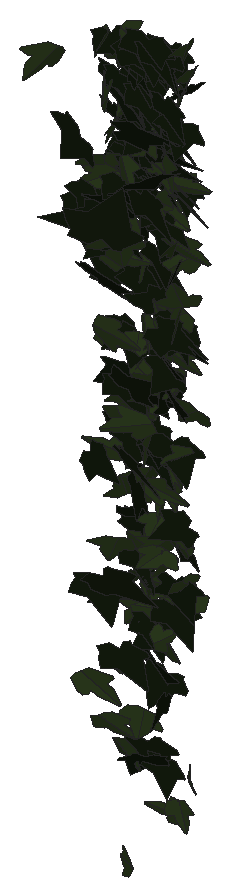
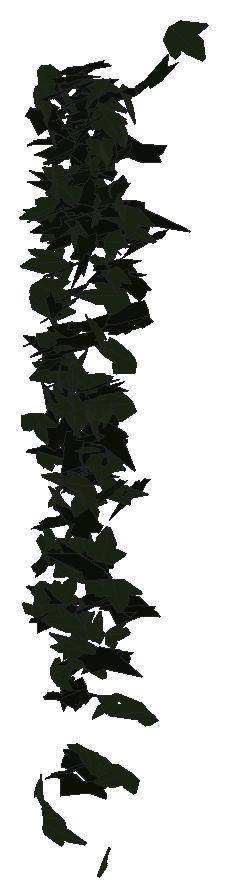
# SketchUp Ruby script. Lengths in millimetres.
U = 1.mm
M = Sketchup.active_model
def pt(a) = Geom::Point3d.new(a.map { |v| v * U })
def face(e, loops, mat)
  f = e.add_face(loops[0].map { |a| pt(a) })
  loops[1..].each { |l| e.add_face(l.map { |a| pt(a) }).erase! }
  f.material = f.back_material = mat if mat
  f
end
# faces: each face lists its corners as indices into pts; further lists are holes
def faces(e, pts, list, mat = nil) = list.each { |f| face(e, (f[0].is_a?(Array) ? f : [f]).map { |l| l.map { |i| pts[i] } }, mat) }
# xy, xz, yz: faces in a plane at the given z, y or x. An outline is a flat list of corners, or four numbers for a rectangle; further outlines are holes
def ring(l) = l.size == 4 ? [[l[0], l[1]], [l[2], l[1]], [l[2], l[3]], [l[0], l[3]]] : l.each_slice(2).to_a
def flat(e, list, mat, &to3) = list.each { |f| face(e, (f[0].is_a?(Array) ? f : [f]).map { |l| ring(l).map { |u, v| to3.(u, v) } }, mat) }
def xy(e, z, list, mat = nil) = flat(e, list, mat) { |x, y| [x, y, z] }
def xz(e, y, list, mat = nil) = flat(e, list, mat) { |x, z| [x, y, z] }
def yz(e, x, list, mat = nil) = flat(e, list, mat) { |y, z| [x, y, z] }
def lines(e, pts, list) = list.each { |a, b| e.add_line(pt(pts[a]), pt(pts[b])) }
# prism: a flat outline (further loops are holes) pulled along v
def prism(e, loops, v, mat = nil)
  f = face(e, loops, mat); d = Geom::Vector3d.new(v.map { |x| x * U })
  f.pushpull(f.normal.samedirection?(d) ? d.length : -d.length)
end
def box(e, o, s, mat = nil) = prism(e, [[o, [o[0] + s[0], o[1], o[2]], [o[0] + s[0], o[1] + s[1], o[2]], [o[0], o[1] + s[1], o[2]]]], [0, 0, s[2]], mat)
def at(x, y, z, deg = 0) = Geom::Transformation.translation(pt([x, y, z])) * Geom::Transformation.rotation(ORIGIN, Z_AXIS, deg.degrees)
def axes(o, x, y, z) = Geom::Transformation.new([*x, 0, *y, 0, *z, 0, *pt(o).to_a, 1])
def part(name) = M.definitions.add(name)
# library, detail: a bought-in or finely detailed component or shape, given as its bounding box
def library(name, o, s) = part(name).tap { |d| box(d.entities, o, s) }
def detail(e, o, s) = box(e.add_group.entities, o, s)
def put(e, d, t, mat = nil) = e.add_instance(d, t).tap { |i| i.material = mat if mat }
def group(e, t, mat = nil) = e.add_group.tap { |g| g.transformation = t; g.material = mat if mat }.entities
root = M.entities
M.materials.add("efeu1").color = [18, 25, 13]
M.materials.add("efeu2").color = [43, 57, 29]
c1 = part("ivyleaf_9")
p = [[39.1,54.8,31.7],[34.5,51.8,30.2],[-5.3,25.2,17.3],[-17.9,28.3,20.9],[-21.6,21.7,17],[-20.2,4.3,5.3],
  [-22.9,-0.3,2.5],[-17.1,-4,-0.6],[-2,-2.1,-1.2],[-0.7,-15.4,-10.1],[16.6,-22.3,-16.7],[21.1,-15.1,-12.5],
  [32.7,-10.7,-11],[46.1,-1.8,-6.6],[30.8,11.2,3.8]]
faces(c1.entities,p,[[0,1,2,3,4,5,6,7,8,9,10,11,12,13,14]],"efeu1")
c2 = part("ivyleaf_10")
p = [[0,12.8,-0.8],[-1.5,51.3,-10.9],[-4.9,51,-11.6],[-13.6,26.5,-7.3],[-13.2,15.9,-4.6],[-21.1,19.3,-7.2],
  [-29.5,16.3,-8.3],[-29.2,8.3,-6.2],[-19.7,-9.8,0.5],[-7.6,-13,4],[1,-12.2,5.8],[-0.4,51.1,-11.1],
  [-1.5,51.1,-10.9],[1,-12.4,5.9],[16.9,-12.4,3.5],[35.1,9.1,-5.1],[35,12.9,-6.1],[20.5,16.4,-4.9],
  [15.8,15,-3.8],[15.3,27.6,-7.1],[12.8,31.3,-7.8]]
faces(c2.entities,p,[[0,1,2,3,4,5,6,7,8,9,10],[11,12,0,13,14,15,16,17,18,19,20]],"efeu2")
put(root,c1,axes([2025,744.4,1522.4],[-0.59045,-0.57511,0.96356],[-0.27948,-0.9703,-0.62642],[2.11729,-0.28846,0.18602]))
put(root,c1,axes([2083.3,733,1360.2],[-1.5486,-0.12856,0.81863],[1.53227,0.14899,0.82363],[-0.3734,1.14456,-0.01526]))
put(root,c2,axes([1950.2,760.7,1650.6],[-0.45254,-0.90858,0.68289],[-0.14048,-0.68385,-0.93556],[2.1586,-0.23498,0.08228]))
put(root,c1,axes([2027.4,832.8,1321.6],[-0.43087,-0.35158,-0.98103],[-1.10797,-0.79,0.41746],[-1.64506,0.62416,-0.02422]))
put(root,c2,axes([2084.4,834.2,963],[-0.61889,-0.15247,0.84845],[-1.00894,-0.67969,-0.32533],[1.29371,-0.60302,0.15216]))
put(root,c2,axes([2044.6,827.3,1294.8],[-1.29698,-0.81371,-0.15005],[0.18292,0.11523,-1.06138],[1.56411,-0.68822,-0.0003]))
put(root,c1,axes([2039.7,842.7,887.6],[1.06306,-0.71655,0.03403],[0.04076,-0.02645,-0.90854],[1.36467,0.55898,0.00063]))
put(root,c1,axes([2094.1,823.6,1427.4],[0.72709,0.98395,0.23303],[0.16081,0.21717,-1.05551],[-1.91772,0.39127,-0.00016]))
put(root,c1,axes([2050.2,864.7,822.7],[0.41731,-0.17934,-0.93924],[1.34399,-0.61934,0.28311],[-1.22702,-0.73937,-0.00933]))
put(root,c1,axes([1950.7,881.2,1323.8],[-0.66445,-0.72966,0.43215],[-0.13711,-0.44014,-0.80134],[1.60814,-0.339,0.11024]))
put(root,c1,axes([2058.5,871,1365.5],[0.5974,-0.8535,-0.21236],[-0.09904,0.20706,-0.90912],[1.67097,0.31741,0.02204]))
put(root,c1,axes([1927.1,869.4,1315.7],[0.29792,-0.80255,-0.41602],[-0.13796,0.40971,-0.81765],[1.71489,0.17239,0.0065]))
put(root,c2,axes([2021.4,870.1,1414.8],[-0.08495,0.88501,-0.17145],[0.01922,-0.17115,-0.88614],[-1.71556,-0.04574,-0.00144]))
put(root,c1,axes([1959.6,881.1,598.4],[-0.64268,-0.70628,-0.39631],[0.3504,0.35119,-0.78275],[1.50099,-0.38439,0.01304]))
put(root,c1,axes([2006.1,877.2,490],[-0.10418,-0.68227,-0.5508],[0.1789,0.54413,-0.68334],[1.65921,-0.10151,0.0391]))
put(root,c2,axes([1964.7,886.5,1077],[-0.06447,0.03819,-0.96645],[1.52583,-0.53985,-0.04943],[-1.02973,-0.80233,-0.01274]))
put(root,c1,axes([1972.1,888.6,1309.1],[1.88697,0.26607,0.22449],[-0.42479,-0.03415,1.02627],[0.50845,-1.016,0.02429]))
put(root,c2,axes([2011,891.6,79.2],[-0.5212,0.5755,0.41446],[0.32636,-0.37737,0.6373],[1.30971,0.32305,0.00613]))
put(root,c2,axes([1932.9,882.9,408.6],[0.95655,0.17501,0.67755],[1.22317,0.21461,-0.53218],[-0.52695,0.81586,-0.00536]))
put(root,c1,axes([1974.9,877.5,616.7],[-0.00616,-0.09918,-0.87578],[0.74471,0.78459,-0.0903],[1.50308,-0.38914,0.04115]))
put(root,c1,axes([1942.5,898,1160.1],[0.00503,-0.4091,0.7989],[1.07046,-0.62183,-0.32029],[1.33122,0.50157,0.25453]))
put(root,c1,axes([1943.4,881,837],[0.55134,-0.5067,-0.76251],[-0.70629,0.66613,-0.58364],[1.59285,0.47076,0.00513]))
put(root,c1,axes([2078.3,903.6,410.2],[-0.26455,0.19758,-0.73243],[0.88609,-0.56567,-0.24095],[-1.13989,-0.48558,-0.01732]))
put(root,c1,axes([1988.6,912.6,1497.6],[-0.39767,-0.43201,0.83597],[0.22129,-0.86162,-0.4162],[1.77719,0.01062,0.23888]))
put(root,c1,axes([1998,896.9,1363.8],[-0.07585,-0.80628,-0.50177],[0.04979,0.50109,-0.80726],[1.8067,-0.04766,0.00118]))
put(root,c1,axes([1971.6,908.8,1244.4],[-1.05319,-0.49747,0.25851],[-0.3625,-0.17479,-0.74411],[1.00351,-0.58524,0.00251]))
put(root,c2,axes([2060.2,897.9,805.6],[0.19964,0.03854,0.74126],[1.38352,0.14594,-0.11046],[-0.28545,0.73428,-0.01695]))
put(root,c1,axes([2039.6,898.7,289.4],[0.44416,0.62056,-0.38436],[-0.26488,-0.3583,-0.66299],[-1.36377,0.2717,0.00359]))
put(root,c2,axes([1984.8,907.6,291.2],[-0.83427,0.37906,-0.48542],[0.68928,-0.32326,-0.57949],[-0.94808,-0.56858,0.00585]))
put(root,c2,axes([2034.4,918,879.4],[0.38125,-0.68078,0.51492],[0.50201,-0.45365,-0.70239],[1.54503,0.31539,0.10116]))
put(root,c1,axes([1991.4,904.1,1452.1],[1.02445,0.21175,-0.63507],[0.98202,0.38797,0.56669],[0.81175,-0.73657,0.11592]))
put(root,c2,axes([1952.6,915.1,1352.3],[0.8859,0.32847,-0.70126],[-1.17258,-0.33857,-0.56755],[-0.89281,0.77059,0.04956]))
put(root,c2,axes([1962.1,891.5,1508.9],[0.44742,-0.28858,0.96722],[-1.10044,0.77551,0.37192],[-1.57456,-0.62399,0.01491]))
put(root,c1,axes([2068.1,918.1,1527.4],[0.35814,-0.82673,0.10934],[0.03484,-0.10797,-0.84786],[1.58676,0.18897,-0.00606]))
put(root,c1,axes([2031.3,919.3,1628.5],[-0.40377,-0.90102,-0.1024],[0.04736,0.09934,-0.92566],[1.7252,-0.2136,0.00145]))
put(root,c2,axes([2094.1,907.8,1272.6],[0.01395,-0.75862,-0.2512],[-0.01958,0.2511,-0.75862],[1.52078,0.01019,-0.00746]))
put(root,c1,axes([2071.2,900.5,1106.8],[0.61999,-0.40309,-0.77176],[-0.09407,0.81412,-0.44608],[1.65442,0.19735,0.26385]))
put(root,c2,axes([1970.1,916.2,835.1],[0.37409,0.13798,0.69312],[-1.09664,-0.38526,0.2401],[0.77877,-0.60879,0.00515]))
put(root,c2,axes([1958.6,928.4,566.7],[-0.29916,-0.20614,0.77495],[0.24086,-0.78618,-0.18346],[1.50705,0.08473,0.18315]))
put(root,c1,axes([2028.9,930.1,857],[-0.15017,-0.48877,0.70375],[0.26647,-0.70458,-0.47365],[1.60879,0.07108,0.14414]))
put(root,c1,axes([2036.5,919.8,1616],[0.44568,-0.82718,-0.10521],[-0.00875,0.10799,-0.85933],[1.58695,0.2329,0.02481]))
put(root,c1,axes([2068.4,931.5,1015.1],[-0.65818,-0.60775,0.4634],[-0.24148,-0.45592,-0.69263],[1.43436,-0.35563,0.09603]))
put(root,c1,axes([2101.4,930.2,731.4],[-0.80179,-0.39468,0.56978],[-0.71924,-0.42814,-0.57599],[1.10581,-0.56464,0.03849]))
put(root,c1,axes([2039.2,932.5,1321.7],[-0.69848,-0.62396,0.42429],[-0.08492,-0.45304,-0.70484],[1.43355,-0.33085,0.16498]))
put(root,c2,axes([2069.8,901.9,1347.5],[-0.08237,0.48159,0.64392],[-0.31237,0.62599,-0.47921],[-1.49813,-0.157,0.06451]))
put(root,c1,axes([1987.6,923.2,954.9],[-0.47855,0.02371,0.8195],[0.88765,-0.70082,0.16338],[1.28324,0.49362,0.1926]))
put(root,c2,axes([1936.8,921,1606.5],[0.53239,-0.8435,0.02444],[0.015,-0.02313,-0.88868],[1.60596,0.27984,0.0002]))
put(root,c2,axes([1941.1,915.8,1377],[-1.12336,-0.66652,-0.1353],[0.18086,0.09656,-0.89027],[1.28169,-0.59781,0.00704]))
put(root,c2,axes([1987.3,920.5,1601.8],[-0.07017,-0.89126,0.02368],[-0.00471,-0.0236,-0.89203],[1.69685,-0.03692,-0.0015]))
put(root,c1,axes([2058,929.1,271.6],[-0.28259,-0.76576,0.05285],[-0.03019,-0.05076,-0.78],[1.46055,-0.14921,-0.0059]))
put(root,c1,axes([1933.8,919,1263.4],[-0.40067,-0.10092,-0.86869],[1.44649,0.42089,-0.23309],[0.82336,-0.78854,-0.01324]))
put(root,c1,axes([2012.5,927.5,1521.6],[0.11998,-0.8391,-0.12858],[-0.00001,0.12893,-0.84142],[1.61562,0.06231,0.00955]))
put(root,c2,axes([2097.8,933.2,866.1],[-0.09863,-0.31934,0.67271],[-0.32182,-0.65167,-0.32238],[1.38021,-0.17477,-0.02709]))
put(root,c2,axes([2083.5,930.4,1127.9],[0.72712,-0.74233,0.4175],[0.46151,-0.34383,-0.83325],[1.55384,0.4495,0.05212]))
put(root,c2,axes([1965,910.8,1209.7],[-0.29853,-0.14478,-0.90391],[1.53988,0.40706,-0.20561],[0.81498,-0.82216,0.05738]))
put(root,c1,axes([1996,917.5,1610.3],[0.30379,-0.61305,-0.58444],[-0.03631,0.59197,-0.62616],[1.61158,0.1289,0.09606]))
put(root,c2,axes([2047.1,929,1403.9],[1.19859,-0.31022,0.57392],[1.01111,-0.21911,-0.70141],[0.72063,0.8234,0.02958]))
put(root,c2,axes([1959.8,923.8,658.2],[-1.07767,-0.593,0.10866],[-0.12819,-0.08591,-0.81986],[1.1402,-0.57014,0.01053]))
put(root,c1,axes([2068.5,936.2,955.5],[0.11624,-0.26606,0.77227],[0.34211,-0.75106,-0.27297],[1.51646,0.18983,0.00239]))
put(root,c1,axes([1965.5,930.4,1539.1],[0.20927,-0.84086,-0.06432],[-0.02125,0.06341,-0.84802],[1.60486,0.11048,-0.00284]))
put(root,c1,axes([2076.4,928.8,881.7],[-0.58486,-0.7536,-0.39936],[0.30652,0.36559,-0.81379],[1.594,-0.34681,0.00995]))
put(root,c2,axes([2048.1,929.5,663.4],[0.98136,0.31871,-0.46657],[-0.75333,-0.24702,-0.60618],[-0.76742,0.65004,-0.0016]))
put(root,c1,axes([2048.7,938.5,1609.9],[-0.87267,-0.67369,0.15156],[-0.07103,-0.15748,-0.81295],[1.31229,-0.45653,0.05678]))
put(root,c1,axes([1950.5,927.1,1609.6],[0.07191,-0.81992,-0.44115],[-0.05258,0.44033,-0.82077],[1.77122,0.04636,-0.00645]))
put(root,c2,axes([2017.6,930.7,1090.2],[-0.10176,0.80361,-0.41174],[0.0647,-0.41038,-0.80536],[-1.71727,-0.06308,-0.00594]))
put(root,c1,axes([2039.6,936.2,1597.6],[0.43029,-0.81824,0.17506],[0.06703,-0.17187,-0.84882],[1.5911,0.22852,-0.01158]))
put(root,c2,axes([2047.1,933.9,682.9],[-0.67321,-0.58412,0.4179],[-0.41833,-0.35544,-0.68287],[1.30132,-0.41644,-0.00333]))
put(root,c2,axes([1956.3,942.6,1283.9],[0.03091,-0.00866,-0.82731],[0.00883,-0.82745,0.00875],[-1.57459,-0.00481,-0.01619]))
put(root,c1,axes([2003,938.7,860.7],[-0.86184,-0.61602,0.09287],[-0.07741,-0.08533,-0.76435],[1.18313,-0.45432,0.01764]))
put(root,c1,axes([2087.2,940.3,1480.8],[-0.58709,-0.78065,0.13568],[-0.06691,-0.13197,-0.83924],[1.50652,-0.31008,0.0156]))
put(root,c2,axes([2015.1,926.3,1590.9],[-0.12042,0.00925,0.89983],[-1.70221,-0.10006,-0.06186],[0.18876,-0.89648,0.01619]))
put(root,c2,axes([2013.4,927.9,1433.5],[1.32658,-0.3506,-0.20457],[-0.32602,0.11448,-0.77985],[0.70039,0.71735,0.02447]))
put(root,c2,axes([1966.3,931.1,1273.6],[1.58491,-0.33134,-0.01417],[-0.02655,0.00326,-0.89626],[0.63063,0.83288,-0.00213]))
put(root,c2,axes([2088.8,934.9,1149],[-1.05884,-0.51743,-0.29505],[-0.41797,-0.1971,0.75976],[-1.05376,0.5981,-0.00488]))
put(root,c1,axes([2043.8,941.2,1020.3],[0.26405,-0.35581,0.72277],[0.4416,-0.68469,-0.3816],[1.46826,0.26991,-0.01521]))
put(root,c2,axes([2016.2,933.8,805.1],[-0.48152,-0.79026,0.19399],[-0.06649,-0.19241,-0.8294],[1.54724,-0.25421,0.02473]))
put(root,c2,axes([2054.5,914.8,509],[0.21693,0.09265,-0.75161],[0.60993,0.68276,0.13276],[1.30588,-0.33429,0.06285]))
put(root,c2,axes([2024.1,938.4,1314.8],[0.01859,-0.73463,0.36837],[0.09093,-0.36727,-0.73369],[1.56143,0.03014,0.03834]))
put(root,c1,axes([1953.8,933.8,1156.7],[-0.82243,-0.66872,0.03372],[0.11131,0.00228,0.79475],[-1.26945,0.43344,0.04784]))
put(root,c1,axes([2024.7,935.9,844.2],[0.50497,-0.75038,-0.0322],[-0.00371,0.03346,-0.79585],[1.42944,0.26517,0.00931]))
put(root,c1,axes([2072.5,935.1,568.4],[-0.15907,-0.80538,-0.37116],[0.06919,0.36938,-0.8097],[1.68632,-0.09113,-0.00179]))
put(root,c2,axes([1997.7,933.6,1050.8],[1.0327,0.47618,-0.15139],[-0.20038,-0.10951,-0.72182],[-0.92962,0.55259,-0.01259]))
put(root,c1,axes([2022.5,946.1,1522.2],[-0.34683,0.04344,0.83239],[-0.47929,-0.81511,-0.0126],[1.51223,-0.24838,0.18692]))
put(root,c1,axes([2049.1,943.3,428.5],[-0.98429,-0.6488,0.02979],[-0.03247,-0.0245,-0.8297],[1.23567,-0.51745,0.00193]))
put(root,c2,axes([2099.5,923.9,696.8],[-0.04122,0.01381,0.77347],[-1.35324,0.30446,-0.02534],[-0.57999,-0.71135,0.00417]))
put(root,c2,axes([2055.8,938.4,791.2],[0.98936,-0.21967,0.46904],[0.80655,-0.20163,-0.56412],[0.56667,0.6705,-0.01597]))
put(root,c1,axes([2032.8,932.5,1343.7],[-1.39461,0.39345,0.13631],[-0.24825,0.04512,-0.83144],[-0.75259,-0.74398,0.02166]))
put(root,c1,axes([2047.3,938.1,1471.3],[0.90425,-0.70325,0.08184],[0.08463,-0.06873,-0.84871],[1.34481,0.47719,-0.00162]))
put(root,c1,axes([2014.9,932.4,1399.9],[0.772,-0.06626,-0.7522],[1.29178,0.40619,0.33024],[0.62981,-0.7519,0.24468]))
put(root,c2,axes([2039.1,937.8,720.6],[1.09753,0.38275,-0.24351],[-0.39031,-0.13135,-0.69213],[-0.77012,0.61205,0.00375]))
put(root,c1,axes([2051,940.5,1076.9],[0.69233,0.01777,-0.7644],[1.45435,0.02044,0.36414],[0.04967,-0.8463,-0.00726]))
put(root,c1,axes([1985,949.3,1042.3],[-0.47984,-0.72096,0.24078],[-0.08064,-0.23995,-0.76286],[1.44438,-0.25291,0.0374]))
put(root,c1,axes([1975.7,952.5,1334.9],[-0.34504,-0.45814,0.65721],[0.05576,-0.67717,-0.46397],[1.52369,-0.07896,0.1658]))
put(root,c1,axes([2017.8,947.6,430.9],[0.20121,-0.22181,0.78729],[0.57698,-0.72667,-0.24544],[1.44582,0.32086,-0.01161]))
put(root,c1,axes([2041.6,934.2,1305.3],[0.26413,-0.65462,-0.50206],[-0.01095,0.50833,-0.6644],[1.57007,0.11367,0.07983]))
put(root,c1,axes([1947.9,949.8,1292.8],[-0.92464,-0.58124,0.26966],[-0.33132,-0.20594,-0.75755],[1.1736,-0.51608,-0.00141]))
put(root,c1,axes([2017.2,947.3,1441.7],[-1.22849,-0.4653,0.11034],[-0.17979,-0.05764,-0.79567],[0.89218,-0.65231,-0.0084]))
put(root,c1,axes([2019.4,953.7,492.8],[0.34667,-0.39016,-0.70402],[0.5217,-0.64861,0.43037],[-1.44032,-0.32884,-0.01356]))
put(root,c2,axes([2075.5,942.2,190.6],[1.10368,-0.24788,0.42428],[0.74309,-0.16605,-0.63066],[0.56783,0.6991,0.00064]))
put(root,c2,axes([1971.3,937.4,894.6],[-1.16044,-0.62896,0.18263],[0.23632,0.13398,0.87599],[-1.22388,0.62224,-0.00402]))
put(root,c2,axes([2002.5,947.8,580.4],[-0.69078,0.24349,0.72411],[0.94915,-0.53178,0.42879],[1.10141,0.61097,0.08463]))
put(root,c1,axes([2039.2,935.1,1385.2],[1.51603,-0.43222,-0.08362],[-0.13699,0.04268,-0.90627],[0.82659,0.79981,0.00317]))
put(root,c2,axes([2050.4,928.9,1316.7],[0.76708,0.48503,0.5669],[0.67907,0.44056,-0.63061],[-1.24702,0.53826,0.00531]))
put(root,c2,axes([2030.9,936.7,973.5],[-1.15201,-0.5947,0.31322],[0.4323,0.21573,0.84855],[-1.20396,0.6465,0.00498]))
put(root,c2,axes([1976.3,939.9,1494.9],[-0.84282,0.63108,-0.3677],[0.41809,-0.29501,-0.7709],[-1.3257,-0.49425,-0.00936]))
put(root,c2,axes([2006.1,935.7,1569.2],[0.39594,0.08406,0.87164],[-1.66312,-0.03797,0.21223],[0.1077,-0.89532,0.07283]))
put(root,c1,axes([2051,955.1,1464.6],[-0.3002,-0.66543,0.51155],[-0.05025,-0.51631,-0.67977],[1.59663,-0.14137,0.07479]))
put(root,c2,axes([1931.3,934.2,309.4],[-1.02876,-0.10909,-0.53123],[0.98976,0.10845,-0.55143],[0.29272,-0.75009,-0.00247]))
put(root,c2,axes([1983.8,944.8,667.9],[-0.10474,0.04318,-0.72069],[1.14668,-0.39551,-0.06971],[-0.75712,-0.60498,-0.00587]))
put(root,c1,axes([2019.2,953,1559.4],[-0.33109,-0.85389,0.14448],[0.02455,-0.1499,-0.87042],[1.64804,-0.16931,0.04199]))
put(root,c1,axes([1965.9,955.3,1044.6],[-0.68022,-0.50814,0.46153],[-0.53026,-0.36817,-0.62111],[1.194,-0.45299,-0.0129]))
put(root,c1,axes([1981.8,938.1,1384.5],[0.97685,-0.53082,-0.30203],[-0.20572,0.30934,-0.72736],[1.14399,0.50889,0.1271]))
put(root,c1,axes([1963.1,944.8,953],[-0.25751,-0.70648,-0.3928],[0.27846,0.37029,-0.71638],[1.51301,-0.18839,0.06499]))
put(root,c2,axes([1961.9,927.9,436.1],[0.05203,0.38404,0.64329],[-0.06335,0.6437,-0.38287],[-1.42448,-0.0146,0.04052]))
put(root,c1,axes([2073.4,958.1,677],[0.86778,-0.43502,-0.60219],[0.83704,-0.41136,0.63018],[-1.13945,-0.63349,0.00432]))
put(root,c1,axes([2025.8,955.9,1208.6],[-0.04771,-0.75344,0.28147],[0.04743,-0.2822,-0.75317],[1.53001,-0.01475,0.03212]))
put(root,c1,axes([2046.4,959.1,1249],[-0.48783,-0.63785,0.44543],[-0.05662,-0.46061,-0.67669],[1.47958,-0.22793,0.12097]))
put(root,c1,axes([2067.2,946.6,608.5],[-0.8578,-0.26509,-0.65886],[1.12778,0.28975,-0.52194],[0.74501,-0.74384,0.03149]))
put(root,c2,axes([1965.8,956.9,1487],[-0.33967,-0.46877,0.64152],[0.23817,-0.66588,-0.45176],[1.49329,-0.00043,0.21797]))
put(root,c1,axes([2012.3,950.5,514],[-0.15166,-0.80622,-0.15795],[0.02284,0.15753,-0.81014],[1.56341,-0.08051,-0.00348]))
put(root,c1,axes([2056.1,951.7,1346],[0.81398,-0.66231,0.33188],[0.35902,-0.27322,-0.78834],[1.36343,0.46735,0.00945]))
put(root,c2,axes([1994.4,946.2,333.8],[1.52645,-0.163,0.05092],[0.0964,-0.00642,-0.81843],[0.31038,0.80363,0.00378]))
put(root,c2,axes([2041.2,955.6,625],[-0.47029,-0.41663,-0.55415],[-0.34489,-0.52903,0.47855],[-1.27361,0.2971,0.07504]))
put(root,c1,axes([2070.1,960.4,1091.9],[-0.53733,-0.77442,0.35747],[-0.23892,-0.33472,-0.82427],[1.60563,-0.30897,-0.00302]))
put(root,c1,axes([2016.5,949.6,1398.2],[0.3371,-0.79812,-0.13693],[-0.05806,0.13349,-0.81754],[1.54008,0.17973,-0.00085]))
put(root,c2,axes([2027.6,957.1,750.2],[-0.09593,-0.3943,0.64119],[0.65355,-0.5839,-0.33207],[1.27482,0.26967,0.21849]))
put(root,c1,axes([1997.3,953.7,1551.3],[-0.30951,-0.80249,-0.07161],[0.02309,0.07061,-0.8188],[1.53319,-0.16306,-0.00212]))
put(root,c2,axes([2047.4,937.8,1082],[-0.48094,0.81695,-0.29826],[-0.20319,0.27911,0.85494],[1.64268,0.27371,0.01843]))
put(root,c1,axes([1996.2,941.1,1407.3],[1.2154,-0.13386,0.59867],[1.13134,-0.07843,-0.65164],[0.28839,0.87182,0.03329]))
put(root,c2,axes([2065.3,943,1042.1],[-1.03242,-0.07339,-0.4915],[0.93745,0.01699,-0.54618],[0.1253,-0.73181,0.03661]))
put(root,c2,axes([1975.5,933.3,1620.1],[-0.08376,0.73505,0.5135],[-0.09947,0.51114,-0.73616],[-1.7036,-0.06598,0.01774]))
put(root,c2,axes([1939.1,949.1,1431.9],[0.32398,-0.85781,0.04092],[-0.00258,-0.04198,-0.87449],[1.63444,0.16997,-0.00949]))
put(root,c1,axes([2015.9,955,1358.3],[0.57233,-0.69775,0.22613],[0.1805,-0.20536,-0.75977],[1.38424,0.31527,0.00557]))
put(root,c1,axes([1997.7,943,684],[-0.68747,0.19357,0.67789],[1.17239,-0.28376,0.40927],[0.6525,0.71379,-0.02114]))
put(root,c1,axes([1947.6,959.9,1492.5],[0.37323,-0.63258,0.51761],[0.22407,-0.50489,-0.66164],[1.53938,0.22687,-0.02919]))
put(root,c2,axes([1993.3,956.5,591.7],[0.27619,-0.18933,-0.69325],[0.80537,-0.54911,0.23855],[-1.10545,-0.44736,0.00059]))
put(root,c2,axes([2068.8,943.8,1252.3],[-1.04719,-0.01152,-0.61627],[1.17121,0.03637,-0.55013],[0.06623,-0.82536,-0.01563]))
put(root,c2,axes([1970.9,957.9,575.1],[-0.13675,-0.58739,-0.48252],[-0.14897,-0.47638,0.59157],[-1.43906,0.10513,-0.01539]))
put(root,c1,axes([1971,944.8,968.4],[0.46464,0.10742,-0.85145],[-1.49547,-0.32795,-0.26668],[-0.65672,0.82281,0.00487]))
put(root,c2,axes([2069.9,946.8,797.7],[-0.39695,0.73523,0.02383],[-0.04011,-0.03073,0.76371],[1.39945,0.20767,0.02865]))
put(root,c1,axes([2002.7,954.4,1593.3],[0.09923,-0.82511,-0.16531],[0.0385,0.16681,-0.82621],[1.6011,0.04713,0.03011]))
put(root,c1,axes([1989,934.3,1559.4],[0.47903,-0.11002,-0.85459],[-0.97305,0.69757,-0.24039],[1.31999,0.55415,0.13293]))
put(root,c1,axes([1977.9,956.6,629.8],[0.11738,-0.85524,-0.10599],[-0.01636,0.10565,-0.85746],[1.64006,0.06226,-0.00097]))
put(root,c1,axes([2053.7,962.3,1073.1],[0.08981,-0.74972,0.31851],[0.17811,-0.31194,-0.74812],[1.54003,0.0798,0.06795]))
put(root,c1,axes([1934.7,955.9,863.5],[0.51623,-0.75607,0.00052],[0.00021,-0.00051,-0.80326],[1.43896,0.27125,-0.00007]))
put(root,c2,axes([1954.8,958.9,736.4],[-0.85535,-0.66729,-0.36218],[-0.29047,-0.33288,0.80271],[-1.4155,0.47154,0.05413]))
put(root,c2,axes([2027.4,945.1,1061.2],[-0.04681,-0.73808,-0.3261],[0.12543,0.32332,-0.73677],[1.53058,-0.04907,0.05041]))
put(root,c1,axes([2011.1,933.3,1281.2],[0.24346,0.11396,-0.8894],[-1.20614,0.64706,-0.00824],[1.20728,0.62347,0.17112]))
put(root,c1,axes([2003.1,949.9,1151.5],[-1.11577,-0.5293,0.18891],[0.26448,0.12797,0.78984],[-1.03639,0.6025,-0.00181]))
put(root,c2,axes([2044.3,948.9,1583.3],[0.92446,-0.75982,-0.29221],[-0.24672,0.26373,-0.90127],[1.52956,0.50177,0.03123]))
put(root,c1,axes([1961.7,947.8,1392.3],[0.61114,-0.6126,-0.45195],[0.10644,0.50817,-0.64907],[1.44494,0.22167,0.23896]))
put(root,c1,axes([2004.5,953.3,280.3],[-0.68541,-0.38511,-0.59413],[0.8395,0.39938,-0.52625],[1.05407,-0.5685,0.03278]))
put(root,c1,axes([1969.4,945.7,698.7],[0.73811,0.00681,0.67598],[1.28657,-0.00902,-0.38775],[0.00843,0.77928,-0.0104]))
put(root,c2,axes([1991.3,956.2,916.7],[0.93136,0.15099,-0.52077],[-0.94485,-0.15732,-0.51212],[-0.41496,0.69709,-0.00278]))
put(root,c2,axes([2071.7,956.2,994.7],[0.73977,-0.61438,0.09714],[0.11283,-0.07743,-0.72697],[1.17843,0.3931,0.00863]))
put(root,c2,axes([2086.7,945.1,616.7],[-0.52727,-0.58567,-0.44141],[0.39381,0.39027,-0.64768],[1.33908,-0.34539,0.01666]))
put(root,c2,axes([2101.2,940.2,694.9],[0.06445,-0.15486,-0.73455],[-0.53753,0.67865,-0.15609],[1.32376,0.28311,-0.02762]))
put(root,c1,axes([1921.9,966.2,1509.3],[0.10379,-0.75642,0.35974],[0.10776,-0.35635,-0.75787],[1.59049,0.07351,0.02787]))
put(root,c2,axes([2088.4,952,569.4],[1.16137,0.41697,0.37283],[-0.6537,-0.15614,0.7368],[0.84019,-0.69785,0.05791]))
put(root,c1,axes([1984,960.6,773.6],[0.40827,-0.24364,0.69908],[0.80944,-0.55518,-0.324],[1.15325,0.47592,-0.02008]))
put(root,c1,axes([1975.6,964,1562],[0.21912,-0.821,0.17555],[0.10369,-0.16952,-0.8285],[1.59449,0.12385,0.02975]))
put(root,c2,axes([1928.8,968.2,1350],[-0.10204,-0.35188,0.74831],[0.29212,-0.74109,-0.33749],[1.54644,0.11677,0.11313]))
put(root,c2,axes([1996.9,959.5,529.5],[-0.94489,-0.4735,0.44751],[-0.53291,-0.35295,-0.68409],[1.1196,-0.56761,0.05206]))
put(root,c1,axes([1987.3,963.2,1583.3],[0.7129,-0.62369,0.43974],[0.42067,-0.38019,-0.72751],[1.39013,0.4349,-0.00536]))
put(root,c2,axes([1947.1,956.3,1017],[-0.66406,0.64965,-0.37007],[0.34587,-0.32245,-0.73739],[-1.38027,-0.39335,-0.00673]))
put(root,c2,axes([2068.7,953.9,166.7],[-0.01643,0.02124,0.74142],[-1.38751,-0.13679,-0.00457],[0.25997,-0.72875,0.02247]))
put(root,c2,axes([1992.6,957,854],[-0.6185,0.07335,-0.64823],[1.10539,-0.29725,-0.32481],[-0.56538,-0.66141,0.07409]))
put(root,c2,axes([1989.1,952.6,535.7],[0.30528,-0.10336,-0.79289],[1.51595,-0.05019,0.16768],[-0.13331,-0.8074,0.09108]))
put(root,c2,axes([1921.3,945.1,1029.5],[-0.20871,-0.17209,-0.79953],[1.3615,0.37077,-0.17793],[0.75435,-0.7168,0.09992]))
put(root,c1,axes([2028.4,950.1,1190.4],[0.76759,-0.54049,-0.43789],[-0.30711,0.41966,-0.66662],[1.28777,0.42224,0.10203]))
put(root,c2,axes([2089.9,957.3,1573.1],[0.00562,-0.85137,0.05429],[0.03399,-0.05421,-0.85119],[1.62326,0.00408,0.01763]))
put(root,c2,axes([1992.3,943.5,989.5],[0.19616,0.77011,0.44627],[0.02124,0.4481,-0.77584],[-1.69386,0.0948,0.04195]))
put(root,c2,axes([1957.5,951.3,1572.7],[-1.187,0.0715,0.54602],[-1.03937,0.02565,-0.62716],[-0.13462,-0.82853,0.02771]))
put(root,c2,axes([1992.1,966.2,909.4],[0.39461,-0.39803,0.60911],[0.67581,-0.49747,-0.44594],[1.20872,0.40808,0.05048]))
put(root,c1,axes([2087.3,960.9,1542.9],[-0.59236,0.48859,-0.5866],[0.24226,-0.59139,-0.56013],[-1.43261,-0.30203,0.14783]))
put(root,c2,axes([2030.1,949.8,954.4],[1.094,-0.32089,0.32932],[-0.49468,0.20812,0.65648],[-0.72186,-0.62893,0.04921]))
put(root,c1,axes([2011.8,971,875],[-0.63903,-0.51469,0.48266],[-0.30808,-0.46408,-0.60748],[1.30707,-0.36102,0.09279]))
put(root,c2,axes([2101.4,953,939.8],[-1.19044,-0.00544,0.43269],[-0.82342,0.02148,-0.62518],[-0.01475,-0.76027,-0.02076]))
put(root,c2,axes([2009.9,944.2,759.7],[-0.04609,0.02425,-0.72519],[-0.59327,0.65487,0.03231],[1.24702,0.31245,-0.01143]))
put(root,c2,axes([2072.9,969.2,1212.1],[-0.71541,-0.43601,0.68517],[-0.39273,-0.67895,-0.54526],[1.49492,-0.38702,0.18465]))
put(root,c2,axes([2067.8,956,1111],[1.04139,0.00407,-0.49725],[-0.93579,0.11483,-0.54012],[0.14132,0.7304,0.08768]))
put(root,c1,axes([1919.9,966.9,1445.1],[0.52858,-0.72908,0.27717],[0.20487,-0.25558,-0.78013],[1.47026,0.29773,0.00905]))
put(root,c2,axes([2037.5,941.8,1420.8],[0.59254,0.45715,-0.77984],[0.88999,0.62441,0.55273],[1.47232,-0.56142,-0.02027]))
put(root,c1,axes([2066.4,968.2,1354.8],[-0.23746,-0.77393,0.1001],[0.01516,-0.10263,-0.78355],[1.48513,-0.12269,0.02401]))
put(root,c2,axes([2057.6,951.6,465.5],[-0.94354,0.53722,-0.37664],[-0.4798,0.27986,0.73101],[1.15282,0.55617,-0.00403]))
put(root,c2,axes([1970.8,945.7,1399.8],[-0.07826,-0.53898,-0.66297],[0.14165,0.65896,-0.54033],[1.61995,-0.08366,0.01522]))
put(root,c1,axes([2050.3,965.3,1174.6],[0.28962,0.40988,0.69617],[-0.45394,-0.65404,0.43722],[1.469,-0.28292,-0.00215]))
put(root,c2,axes([2078.7,957.9,1618.2],[-0.12724,-0.82828,-0.08372],[0.05176,0.08177,-0.83072],[1.58357,-0.06922,0.02042]))
put(root,c1,axes([2037.1,968.1,923.9],[0.46863,0.31078,0.78856],[-0.91442,-0.6253,0.39647],[1.32892,-0.53986,-0.00527]))
put(root,c1,axes([1986.6,939.2,1415.2],[0.24543,0.35513,0.7991],[0.45635,0.76242,-0.37752],[-1.60048,0.27185,0.0149]))
put(root,c1,axes([1982.1,972.4,1315.2],[0.14294,-0.51258,0.6061],[0.2157,-0.59564,-0.51778],[1.49525,0.13493,0.01675]))
put(root,c2,axes([2056.6,954.7,1431.9],[0.05557,-0.79802,-0.29345],[0.07781,0.2946,-0.79708],[1.61634,0.01325,0.04846]))
put(root,c1,axes([2021.3,958,1117],[-1.21625,-0.58234,0.19141],[0.29184,0.11584,0.86442],[-1.12955,0.65697,0.01725]))
put(root,c1,axes([1970.3,963.2,1397],[-0.57898,-0.72268,-0.38636],[0.27746,0.35783,-0.78409],[1.53475,-0.33732,-0.004]))
put(root,c2,axes([2026.3,961.1,1411.5],[1.32851,0.27879,-0.29682],[-0.54969,-0.07628,-0.7509],[-0.54634,0.75468,0.03375]))
put(root,c1,axes([1966.8,962.9,1375.8],[-0.94507,-0.45951,-0.41466],[0.54069,0.30309,-0.67609],[1.04656,-0.57154,-0.02515]))
put(root,c2,axes([1980.3,961.9,991.1],[0.43513,-0.70155,0.04792],[0.00136,-0.05016,-0.73772],[1.3383,0.22815,-0.01483]))
put(root,c1,axes([2041.3,967.1,1598],[0.05067,-0.84739,-0.0878],[-0.00297,0.0878,-0.84781],[1.62138,0.02664,0.00119]))
put(root,c2,axes([1955.6,957.1,916.6],[-0.84744,-0.55203,-0.14254],[0.17193,0.11026,-0.70922],[1.07136,-0.45434,0.00107]))
put(root,c1,axes([1975.3,969.7,1463.8],[0.44116,-0.75724,0.24907],[0.19538,-0.22887,-0.79136],[1.5045,0.25177,0.02974]))
put(root,c1,axes([2007.9,963.2,1459.6],[0.43599,-0.75036,-0.18724],[0.02347,0.1988,-0.7816],[1.47168,0.21913,0.06793]))
put(root,c2,axes([2006.8,961.7,579.6],[0.72439,-0.01616,0.7818],[1.48823,0.01005,-0.38049],[-0.00374,0.86947,0.01892]))
put(root,c1,axes([2040.7,972.4,1098.3],[-0.55341,-0.72484,0.15526],[-0.06932,-0.1526,-0.78067],[1.40911,-0.29218,0.02257]))
put(root,c2,axes([1956.6,972.9,1001.2],[-0.05041,-0.45044,0.65683],[0.66033,-0.59808,-0.39616],[1.3644,0.27281,0.216]))
put(root,c2,axes([2036.9,971.6,1056.2],[0.39053,-0.48673,0.64315],[0.81845,-0.49542,-0.51213],[1.29866,0.45859,0.12936]))
put(root,c2,axes([2098.6,948.1,241.4],[-0.29383,0.152,0.68158],[-0.84231,0.51865,-0.21592],[-1.02805,-0.46839,-0.0179]))
put(root,c2,axes([2065.5,965.9,1525.3],[0.60935,-0.74024,0.1502],[0.18079,-0.12238,-0.80562],[1.42611,0.3318,0.03795]))
put(root,c1,axes([1955.4,971.3,547.8],[0.02897,0.0354,-0.79946],[-0.36859,-0.77567,-0.03804],[-1.47774,0.19417,-0.00619]))
put(root,c1,axes([2034.2,962.6,1347],[1.06656,-0.56093,-0.02549],[-0.03166,0.01942,-0.7929],[1.06819,0.56065,0.00196]))
put(root,c1,axes([1991.3,951.3,930.9],[1.42563,0.35719,-0.05557],[-0.09791,-0.02122,-0.82987],[-0.68098,0.75083,0.00298]))
put(root,c2,axes([1975.4,960.7,1172.2],[0.95422,-0.62547,-0.22873],[-0.27666,0.17662,-0.80161],[1.23693,0.52202,-0.00284]))
put(root,c2,axes([1942.6,968.7,1523.6],[0.29522,-0.7754,0.28206],[0.1822,-0.26815,-0.78981],[1.55975,0.17809,0.03887]))
put(root,c2,axes([2068.8,948.6,1358.9],[-0.45215,-0.29741,-0.81773],[1.03843,0.60938,-0.38016],[1.29001,-0.59479,0.01941]))
